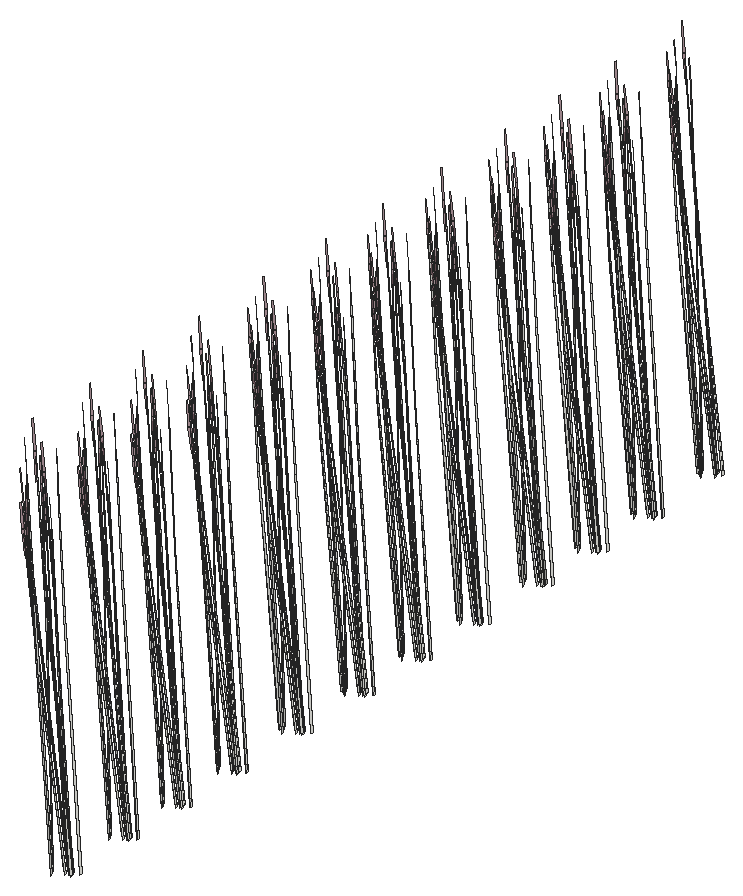
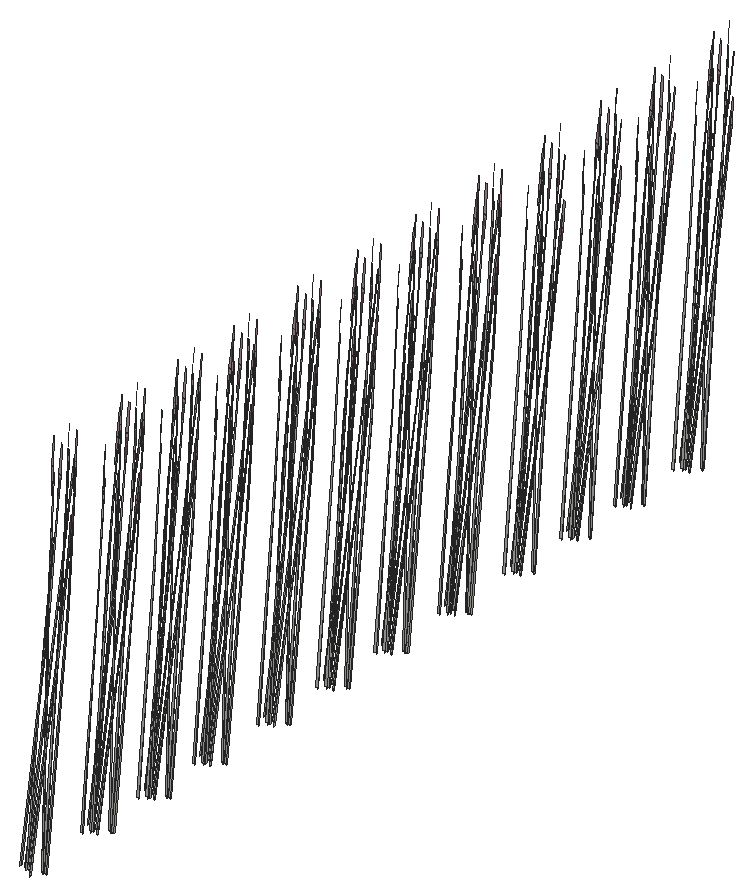
# SketchUp Ruby script. Lengths in inches.
U = 1.inch
M = Sketchup.active_model
def pt(a) = Geom::Point3d.new(a.map { |v| v * U })
def face(e, loops, mat)
  f = e.add_face(loops[0].map { |a| pt(a) })
  loops[1..].each { |l| e.add_face(l.map { |a| pt(a) }).erase! }
  f.material = f.back_material = mat if mat
  f
end
# faces: each face lists its corners as indices into pts; further lists are holes
def faces(e, pts, list, mat = nil) = list.each { |f| face(e, (f[0].is_a?(Array) ? f : [f]).map { |l| l.map { |i| pts[i] } }, mat) }
# xy, xz, yz: faces in a plane at the given z, y or x. An outline is a flat list of corners, or four numbers for a rectangle; further outlines are holes
def ring(l) = l.size == 4 ? [[l[0], l[1]], [l[2], l[1]], [l[2], l[3]], [l[0], l[3]]] : l.each_slice(2).to_a
def flat(e, list, mat, &to3) = list.each { |f| face(e, (f[0].is_a?(Array) ? f : [f]).map { |l| ring(l).map { |u, v| to3.(u, v) } }, mat) }
def xy(e, z, list, mat = nil) = flat(e, list, mat) { |x, y| [x, y, z] }
def xz(e, y, list, mat = nil) = flat(e, list, mat) { |x, z| [x, y, z] }
def yz(e, x, list, mat = nil) = flat(e, list, mat) { |y, z| [x, y, z] }
def lines(e, pts, list) = list.each { |a, b| e.add_line(pt(pts[a]), pt(pts[b])) }
# prism: a flat outline (further loops are holes) pulled along v
def prism(e, loops, v, mat = nil)
  f = face(e, loops, mat); d = Geom::Vector3d.new(v.map { |x| x * U })
  f.pushpull(f.normal.samedirection?(d) ? d.length : -d.length)
end
def box(e, o, s, mat = nil) = prism(e, [[o, [o[0] + s[0], o[1], o[2]], [o[0] + s[0], o[1] + s[1], o[2]], [o[0], o[1] + s[1], o[2]]]], [0, 0, s[2]], mat)
def at(x, y, z, deg = 0) = Geom::Transformation.translation(pt([x, y, z])) * Geom::Transformation.rotation(ORIGIN, Z_AXIS, deg.degrees)
def axes(o, x, y, z) = Geom::Transformation.new([*x, 0, *y, 0, *z, 0, *pt(o).to_a, 1])
def part(name) = M.definitions.add(name)
# library, detail: a bought-in or finely detailed component or shape, given as its bounding box
def library(name, o, s) = part(name).tap { |d| box(d.entities, o, s) }
def detail(e, o, s) = box(e.add_group.entities, o, s)
def put(e, d, t, mat = nil) = e.add_instance(d, t).tap { |i| i.material = mat if mat }
def group(e, t, mat = nil) = e.add_group.tap { |g| g.transformation = t; g.material = mat if mat }.entities
root = M.entities
M.materials.add("LightPink_Translucent").color = [144, 107, 117]
M.materials["LightPink_Translucent"].alpha = 0.75
c1 = part("blade")
p = [[2.15,0.21,22],[0,0.17,0],[0.09,0.45,0],[2.18,0.31,22],[2.29,0.31,22],[0.38,0.45,0],
  [2.48,0.24,33],[2.49,0.24,33],[2.48,0.22,33]]
faces(c1.entities,p,[[0,1,2,3],[4,5,2,3],[6,3,4,7],[8,0,3,6]])
c2 = part("seeds")
p = [[0.3,-0.1,1.38],[-0.01,-0.03,1.59],[-0.01,-0.03,0.03],[0.14,-0.07,-0.07],[0.29,-0.03,3],[0.15,0.01,3.11]]
faces(c2.entities,p,[[0,1,2,3],[1,0,4,5]],"LightPink_Translucent")
c3 = part("blade with seeds")
put(c3.entities,c1,at(0,0,0))
put(c3.entities,c2,axes([2.4,0.25,30.99],[1.5799,-0.05474,1.17369],[-0.12525,1.92788,0.29478],[-0.07173,-0.02425,1.56792]))
put(root,c3,axes([331.78,276.37,49.78],[0,-0.39075,-0.43871],[0.56491,0,0],[0,-0.089,1.3917]))
put(root,c3,axes([332.125,276.55,50.06],[-0.46965,0.32852,0.27176],[-0.46994,-0.32506,-0.32244],[-0.0164,-0.09329,1.45692]))
put(root,c3,axes([333.4,277.23,50.16],[0.13383,-0.46302,-0.20702],[0.63453,0.08071,0.45303],[-0.11087,-0.06394,1.38231]))
put(root,c3,axes([332.02,276.73,50.19],[0,0.39075,0.43871],[-0.56491,0,0],[0,-0.089,1.3917]))
put(root,c3,axes([333.35,277.05,49.95],[-0.30332,-0.32798,-0.39531],[0.45944,-0.23096,0.19025],[-0.09816,-0.04058,1.26923]))
put(root,c3,axes([332.52,277.77,49.79],[-0.11861,-0.34048,-0.27372],[0.47106,-0.09668,0.27372],[-0.09497,-0.03926,1.22797]))
put(root,c3,axes([333.63,277.34,50.3125],[-0.09741,0.34873,0.12794],[-0.4759,-0.06053,-0.36534],[-0.08661,-0.03581,1.11991]))
put(root,c3,axes([334.25,277.35,50.18],[-0.49304,-0.31451,-0.2226],[0.41487,-0.35316,0.48713],[-0.13277,0.03679,1.48635]))
put(root,c3,axes([332.95,277.95,50.19],[0.47255,0.19538,0.43871],[-0.28245,0.35034,0],[-0.10763,-0.0445,1.3917]))
put(root,c3,axes([334,277.28,49.95],[-0.54829,0.02412,-0.39531],[-0.04958,-0.40041,0.19025],[-0.09816,0.04058,1.26923]))
put(root,c3,axes([334.02,277.51,49.82],[-0.34009,0.2937,-0.55095],[-0.42248,-0.26632,-0.1446],[-0.13628,0.07327,1.21613]))
put(root,c3,axes([334.58,278.31,49.78],[-0.47255,0.19538,-0.43871],[-0.28245,-0.35034,0],[-0.10763,0.0445,1.3917]))
put(root,c3,axes([331.78,286.17,49.78],[0,-0.39075,-0.43871],[0.56491,0,0],[0,-0.089,1.3917]))
put(root,c3,axes([332.125,286.35,50.06],[-0.46965,0.32852,0.27176],[-0.46994,-0.32506,-0.32244],[-0.0164,-0.09329,1.45692]))
put(root,c3,axes([333.4,287.04,50.16],[0.13383,-0.46302,-0.20702],[0.63453,0.08071,0.45303],[-0.11087,-0.06394,1.38231]))
put(root,c3,axes([332.02,286.53,50.19],[0,0.39075,0.43871],[-0.56491,0,0],[0,-0.089,1.3917]))
put(root,c3,axes([333.35,286.85,49.95],[-0.30332,-0.32798,-0.39531],[0.45944,-0.23096,0.19025],[-0.09816,-0.04058,1.26923]))
put(root,c3,axes([332.52,287.58,49.79],[-0.11861,-0.34048,-0.27372],[0.47106,-0.09668,0.27372],[-0.09497,-0.03926,1.22797]))
put(root,c3,axes([333.63,287.15,50.3125],[-0.09741,0.34873,0.12794],[-0.4759,-0.06053,-0.36534],[-0.08661,-0.03581,1.11991]))
put(root,c3,axes([334.25,287.15,50.18],[-0.49304,-0.31451,-0.2226],[0.41487,-0.35316,0.48713],[-0.13277,0.03679,1.48635]))
put(root,c3,axes([332.95,287.75,50.19],[0.47255,0.19538,0.43871],[-0.28245,0.35034,0],[-0.10763,-0.0445,1.3917]))
put(root,c3,axes([334,287.08,49.95],[-0.54829,0.02412,-0.39531],[-0.04958,-0.40041,0.19025],[-0.09816,0.04058,1.26923]))
put(root,c3,axes([334.02,287.32,49.82],[-0.34009,0.2937,-0.55095],[-0.42248,-0.26632,-0.1446],[-0.13628,0.07327,1.21613]))
put(root,c3,axes([334.58,288.12,49.78],[-0.47255,0.19538,-0.43871],[-0.28245,-0.35034,0],[-0.10763,0.0445,1.3917]))
put(root,c3,axes([331.78,295.15,49.78],[0,-0.39075,-0.43871],[0.56491,0,0],[0,-0.089,1.3917]))
put(root,c3,axes([332.125,295.33,50.06],[-0.46965,0.32852,0.27176],[-0.46994,-0.32506,-0.32244],[-0.0164,-0.09329,1.45692]))
put(root,c3,axes([333.4,296.01,50.16],[0.13383,-0.46302,-0.20702],[0.63453,0.08071,0.45303],[-0.11087,-0.06394,1.38231]))
put(root,c3,axes([332.02,295.51,50.19],[0,0.39075,0.43871],[-0.56491,0,0],[0,-0.089,1.3917]))
put(root,c3,axes([333.35,295.82,49.95],[-0.30332,-0.32798,-0.39531],[0.45944,-0.23096,0.19025],[-0.09816,-0.04058,1.26923]))
put(root,c3,axes([332.52,296.55,49.79],[-0.11861,-0.34048,-0.27372],[0.47106,-0.09668,0.27372],[-0.09497,-0.03926,1.22797]))
put(root,c3,axes([333.63,296.12,50.3125],[-0.09741,0.34873,0.12794],[-0.4759,-0.06053,-0.36534],[-0.08661,-0.03581,1.11991]))
put(root,c3,axes([334.25,296.13,50.18],[-0.49304,-0.31451,-0.2226],[0.41487,-0.35316,0.48713],[-0.13277,0.03679,1.48635]))
put(root,c3,axes([332.95,296.73,50.19],[0.47255,0.19538,0.43871],[-0.28245,0.35034,0],[-0.10763,-0.0445,1.3917]))
put(root,c3,axes([334,296.06,49.95],[-0.54829,0.02412,-0.39531],[-0.04958,-0.40041,0.19025],[-0.09816,0.04058,1.26923]))
put(root,c3,axes([334.02,296.29,49.82],[-0.34009,0.2937,-0.55095],[-0.42248,-0.26632,-0.1446],[-0.13628,0.07327,1.21613]))
put(root,c3,axes([334.58,297.09,49.78],[-0.47255,0.19538,-0.43871],[-0.28245,-0.35034,0],[-0.10763,0.0445,1.3917]))
put(root,c3,axes([331.78,304.63,49.78],[0,-0.39075,-0.43871],[0.56491,0,0],[0,-0.089,1.3917]))
put(root,c3,axes([332.125,304.8125,50.06],[-0.46965,0.32852,0.27176],[-0.46994,-0.32506,-0.32244],[-0.0164,-0.09329,1.45692]))
put(root,c3,axes([333.4,305.5,50.16],[0.13383,-0.46302,-0.20702],[0.63453,0.08071,0.45303],[-0.11087,-0.06394,1.38231]))
put(root,c3,axes([332.02,304.99,50.19],[0,0.39075,0.43871],[-0.56491,0,0],[0,-0.089,1.3917]))
put(root,c3,axes([333.35,305.31,49.95],[-0.30332,-0.32798,-0.39531],[0.45944,-0.23096,0.19025],[-0.09816,-0.04058,1.26923]))
put(root,c3,axes([332.52,306.04,49.79],[-0.11861,-0.34048,-0.27372],[0.47106,-0.09668,0.27372],[-0.09497,-0.03926,1.22797]))
put(root,c3,axes([333.63,305.61,50.3125],[-0.09741,0.34873,0.12794],[-0.4759,-0.06053,-0.36534],[-0.08661,-0.03581,1.11991]))
put(root,c3,axes([334.25,305.61,50.18],[-0.49304,-0.31451,-0.2226],[0.41487,-0.35316,0.48713],[-0.13277,0.03679,1.48635]))
put(root,c3,axes([332.95,306.21,50.19],[0.47255,0.19538,0.43871],[-0.28245,0.35034,0],[-0.10763,-0.0445,1.3917]))
put(root,c3,axes([334,305.54,49.95],[-0.54829,0.02412,-0.39531],[-0.04958,-0.40041,0.19025],[-0.09816,0.04058,1.26923]))
put(root,c3,axes([334.02,305.78,49.82],[-0.34009,0.2937,-0.55095],[-0.42248,-0.26632,-0.1446],[-0.13628,0.07327,1.21613]))
put(root,c3,axes([334.58,306.58,49.78],[-0.47255,0.19538,-0.43871],[-0.28245,-0.35034,0],[-0.10763,0.0445,1.3917]))
put(root,c3,axes([331.78,315.62,49.78],[0,-0.39075,-0.43871],[0.56491,0,0],[0,-0.089,1.3917]))
put(root,c3,axes([331.64,315.92,50.1],[-0.63136,0,0],[0,-0.43672,-0.456],[0,-0.09947,1.44655]))
put(root,c3,axes([332.125,315.8,50.06],[-0.46965,0.32852,0.27176],[-0.46994,-0.32506,-0.32244],[-0.0164,-0.09329,1.45692]))
put(root,c3,axes([333.4,316.49,50.16],[0.13383,-0.46302,-0.20702],[0.63453,0.08071,0.45303],[-0.11087,-0.06394,1.38231]))
put(root,c3,axes([332.02,315.98,50.19],[0,0.39075,0.43871],[-0.56491,0,0],[0,-0.089,1.3917]))
put(root,c3,axes([333.35,316.3,49.95],[-0.30332,-0.32798,-0.39531],[0.45944,-0.23096,0.19025],[-0.09816,-0.04058,1.26923]))
put(root,c3,axes([332.52,317.03,49.79],[-0.11861,-0.34048,-0.27372],[0.47106,-0.09668,0.27372],[-0.09497,-0.03926,1.22797]))
put(root,c3,axes([333.63,316.6,50.3125],[-0.09741,0.34873,0.12794],[-0.4759,-0.06053,-0.36534],[-0.08661,-0.03581,1.11991]))
put(root,c3,axes([334.25,316.6,50.18],[-0.49304,-0.31451,-0.2226],[0.41487,-0.35316,0.48713],[-0.13277,0.03679,1.48635]))
put(root,c3,axes([332.95,317.2,50.19],[0.47255,0.19538,0.43871],[-0.28245,0.35034,0],[-0.10763,-0.0445,1.3917]))
put(root,c3,axes([334,316.53,49.95],[-0.54829,0.02412,-0.39531],[-0.04958,-0.40041,0.19025],[-0.09816,0.04058,1.26923]))
put(root,c3,axes([334.02,316.77,49.82],[-0.34009,0.2937,-0.55095],[-0.42248,-0.26632,-0.1446],[-0.13628,0.07327,1.21613]))
put(root,c3,axes([334.58,317.57,49.78],[-0.47255,0.19538,-0.43871],[-0.28245,-0.35034,0],[-0.10763,0.0445,1.3917]))
put(root,c3,axes([331.78,326.22,49.78],[0,-0.39075,-0.43871],[0.56491,0,0],[0,-0.089,1.3917]))
put(root,c3,axes([331.64,326.51,50.1],[-0.63136,0,0],[0,-0.43672,-0.456],[0,-0.09947,1.44655]))
put(root,c3,axes([332.125,326.4,50.06],[-0.46965,0.32852,0.27176],[-0.46994,-0.32506,-0.32244],[-0.0164,-0.09329,1.45692]))
put(root,c3,axes([333.4,327.08,50.16],[0.13383,-0.46302,-0.20702],[0.63453,0.08071,0.45303],[-0.11087,-0.06394,1.38231]))
put(root,c3,axes([332.02,326.58,50.19],[0,0.39075,0.43871],[-0.56491,0,0],[0,-0.089,1.3917]))
put(root,c3,axes([333.35,326.9,49.95],[-0.30332,-0.32798,-0.39531],[0.45944,-0.23096,0.19025],[-0.09816,-0.04058,1.26923]))
put(root,c3,axes([332.52,327.625,49.79],[-0.11861,-0.34048,-0.27372],[0.47106,-0.09668,0.27372],[-0.09497,-0.03926,1.22797]))
put(root,c3,axes([333.63,327.19,50.3125],[-0.09741,0.34873,0.12794],[-0.4759,-0.06053,-0.36534],[-0.08661,-0.03581,1.11991]))
put(root,c3,axes([334.25,327.2,50.18],[-0.49304,-0.31451,-0.2226],[0.41487,-0.35316,0.48713],[-0.13277,0.03679,1.48635]))
put(root,c3,axes([332.95,327.8,50.19],[0.47255,0.19538,0.43871],[-0.28245,0.35034,0],[-0.10763,-0.0445,1.3917]))
put(root,c3,axes([334,327.13,49.95],[-0.54829,0.02412,-0.39531],[-0.04958,-0.40041,0.19025],[-0.09816,0.04058,1.26923]))
put(root,c3,axes([334.02,327.36,49.82],[-0.34009,0.2937,-0.55095],[-0.42248,-0.26632,-0.1446],[-0.13628,0.07327,1.21613]))
put(root,c3,axes([334.58,328.16,49.78],[-0.47255,0.19538,-0.43871],[-0.28245,-0.35034,0],[-0.10763,0.0445,1.3917]))
put(root,c3,axes([331.78,335.92,49.78],[0,-0.39075,-0.43871],[0.56491,0,0],[0,-0.089,1.3917]))
put(root,c3,axes([331.64,336.22,50.1],[-0.63136,0,0],[0,-0.43672,-0.456],[0,-0.09947,1.44655]))
put(root,c3,axes([332.125,336.1,50.06],[-0.46965,0.32852,0.27176],[-0.46994,-0.32506,-0.32244],[-0.0164,-0.09329,1.45692]))
put(root,c3,axes([333.4,336.79,50.16],[0.13383,-0.46302,-0.20702],[0.63453,0.08071,0.45303],[-0.11087,-0.06394,1.38231]))
put(root,c3,axes([332.02,336.29,50.19],[0,0.39075,0.43871],[-0.56491,0,0],[0,-0.089,1.3917]))
put(root,c3,axes([333.35,336.6,49.95],[-0.30332,-0.32798,-0.39531],[0.45944,-0.23096,0.19025],[-0.09816,-0.04058,1.26923]))
put(root,c3,axes([332.52,337.33,49.79],[-0.11861,-0.34048,-0.27372],[0.47106,-0.09668,0.27372],[-0.09497,-0.03926,1.22797]))
put(root,c3,axes([333.63,336.9,50.3125],[-0.09741,0.34873,0.12794],[-0.4759,-0.06053,-0.36534],[-0.08661,-0.03581,1.11991]))
put(root,c3,axes([334.25,336.9,50.18],[-0.49304,-0.31451,-0.2226],[0.41487,-0.35316,0.48713],[-0.13277,0.03679,1.48635]))
put(root,c3,axes([332.95,337.51,50.19],[0.47255,0.19538,0.43871],[-0.28245,0.35034,0],[-0.10763,-0.0445,1.3917]))
put(root,c3,axes([334,336.84,49.95],[-0.54829,0.02412,-0.39531],[-0.04958,-0.40041,0.19025],[-0.09816,0.04058,1.26923]))
put(root,c3,axes([334.02,337.07,49.82],[-0.34009,0.2937,-0.55095],[-0.42248,-0.26632,-0.1446],[-0.13628,0.07327,1.21613]))
put(root,c3,axes([334.58,337.87,49.78],[-0.47255,0.19538,-0.43871],[-0.28245,-0.35034,0],[-0.10763,0.0445,1.3917]))
put(root,c3,axes([331.78,345.86,49.78],[0,-0.39075,-0.43871],[0.56491,0,0],[0,-0.089,1.3917]))
put(root,c3,axes([331.64,346.15,50.1],[-0.63136,0,0],[0,-0.43672,-0.456],[0,-0.09947,1.44655]))
put(root,c3,axes([332.125,346.04,50.06],[-0.46965,0.32852,0.27176],[-0.46994,-0.32506,-0.32244],[-0.0164,-0.09329,1.45692]))
put(root,c3,axes([333.4,346.72,50.16],[0.13383,-0.46302,-0.20702],[0.63453,0.08071,0.45303],[-0.11087,-0.06394,1.38231]))
put(root,c3,axes([332.02,346.22,50.19],[0,0.39075,0.43871],[-0.56491,0,0],[0,-0.089,1.3917]))
put(root,c3,axes([333.35,346.54,49.95],[-0.30332,-0.32798,-0.39531],[0.45944,-0.23096,0.19025],[-0.09816,-0.04058,1.26923]))
put(root,c3,axes([332.52,347.26,49.79],[-0.11861,-0.34048,-0.27372],[0.47106,-0.09668,0.27372],[-0.09497,-0.03926,1.22797]))
put(root,c3,axes([333.63,346.83,50.3125],[-0.09741,0.34873,0.12794],[-0.4759,-0.06053,-0.36534],[-0.08661,-0.03581,1.11991]))
put(root,c3,axes([334.25,346.84,50.18],[-0.49304,-0.31451,-0.2226],[0.41487,-0.35316,0.48713],[-0.13277,0.03679,1.48635]))
put(root,c3,axes([332.95,347.44,50.19],[0.47255,0.19538,0.43871],[-0.28245,0.35034,0],[-0.10763,-0.0445,1.3917]))
put(root,c3,axes([334,346.77,49.95],[-0.54829,0.02412,-0.39531],[-0.04958,-0.40041,0.19025],[-0.09816,0.04058,1.26923]))
put(root,c3,axes([334.02,347,49.82],[-0.34009,0.2937,-0.55095],[-0.42248,-0.26632,-0.1446],[-0.13628,0.07327,1.21613]))
put(root,c3,axes([334.58,347.8,49.78],[-0.47255,0.19538,-0.43871],[-0.28245,-0.35034,0],[-0.10763,0.0445,1.3917]))
put(root,c3,axes([331.78,356.58,49.78],[0,-0.39075,-0.43871],[0.56491,0,0],[0,-0.089,1.3917]))
put(root,c3,axes([331.64,356.875,50.1],[-0.63136,0,0],[0,-0.43672,-0.456],[0,-0.09947,1.44655]))
put(root,c3,axes([332.125,356.76,50.06],[-0.46965,0.32852,0.27176],[-0.46994,-0.32506,-0.32244],[-0.0164,-0.09329,1.45692]))
put(root,c3,axes([333.4,357.45,50.16],[0.13383,-0.46302,-0.20702],[0.63453,0.08071,0.45303],[-0.11087,-0.06394,1.38231]))
put(root,c3,axes([332.02,356.94,50.19],[0,0.39075,0.43871],[-0.56491,0,0],[0,-0.089,1.3917]))
put(root,c3,axes([333.35,357.26,49.95],[-0.30332,-0.32798,-0.39531],[0.45944,-0.23096,0.19025],[-0.09816,-0.04058,1.26923]))
put(root,c3,axes([332.52,357.99,49.79],[-0.11861,-0.34048,-0.27372],[0.47106,-0.09668,0.27372],[-0.09497,-0.03926,1.22797]))
put(root,c3,axes([333.63,357.56,50.3125],[-0.09741,0.34873,0.12794],[-0.4759,-0.06053,-0.36534],[-0.08661,-0.03581,1.11991]))
put(root,c3,axes([334.25,357.56,50.18],[-0.49304,-0.31451,-0.2226],[0.41487,-0.35316,0.48713],[-0.13277,0.03679,1.48635]))
put(root,c3,axes([332.95,358.16,50.19],[0.47255,0.19538,0.43871],[-0.28245,0.35034,0],[-0.10763,-0.0445,1.3917]))
put(root,c3,axes([334,357.49,49.95],[-0.54829,0.02412,-0.39531],[-0.04958,-0.40041,0.19025],[-0.09816,0.04058,1.26923]))
put(root,c3,axes([334.02,357.73,49.82],[-0.34009,0.2937,-0.55095],[-0.42248,-0.26632,-0.1446],[-0.13628,0.07327,1.21613]))
put(root,c3,axes([334.58,358.53,49.78],[-0.47255,0.19538,-0.43871],[-0.28245,-0.35034,0],[-0.10763,0.0445,1.3917]))
put(root,c3,axes([331.78,365.91,49.78],[0,-0.39075,-0.43871],[0.56491,0,0],[0,-0.089,1.3917]))
put(root,c3,axes([331.64,366.2,50.1],[-0.63136,0,0],[0,-0.43672,-0.456],[0,-0.09947,1.44655]))
put(root,c3,axes([332.125,366.09,50.06],[-0.46965,0.32852,0.27176],[-0.46994,-0.32506,-0.32244],[-0.0164,-0.09329,1.45692]))
put(root,c3,axes([333.4,366.77,50.16],[0.13383,-0.46302,-0.20702],[0.63453,0.08071,0.45303],[-0.11087,-0.06394,1.38231]))
put(root,c3,axes([332.02,366.27,50.19],[0,0.39075,0.43871],[-0.56491,0,0],[0,-0.089,1.3917]))
put(root,c3,axes([333.35,366.58,49.95],[-0.30332,-0.32798,-0.39531],[0.45944,-0.23096,0.19025],[-0.09816,-0.04058,1.26923]))
put(root,c3,axes([332.52,367.3125,49.79],[-0.11861,-0.34048,-0.27372],[0.47106,-0.09668,0.27372],[-0.09497,-0.03926,1.22797]))
put(root,c3,axes([333.63,366.88,50.3125],[-0.09741,0.34873,0.12794],[-0.4759,-0.06053,-0.36534],[-0.08661,-0.03581,1.11991]))
put(root,c3,axes([334.25,366.89,50.18],[-0.49304,-0.31451,-0.2226],[0.41487,-0.35316,0.48713],[-0.13277,0.03679,1.48635]))
put(root,c3,axes([332.95,367.49,50.19],[0.47255,0.19538,0.43871],[-0.28245,0.35034,0],[-0.10763,-0.0445,1.3917]))
put(root,c3,axes([334,366.82,49.95],[-0.54829,0.02412,-0.39531],[-0.04958,-0.40041,0.19025],[-0.09816,0.04058,1.26923]))
put(root,c3,axes([334.02,367.05,49.82],[-0.34009,0.2937,-0.55095],[-0.42248,-0.26632,-0.1446],[-0.13628,0.07327,1.21613]))
put(root,c3,axes([334.58,367.85,49.78],[-0.47255,0.19538,-0.43871],[-0.28245,-0.35034,0],[-0.10763,0.0445,1.3917]))
put(root,c3,axes([331.78,375.38,49.78],[0,-0.39075,-0.43871],[0.56491,0,0],[0,-0.089,1.3917]))
put(root,c3,axes([331.64,375.67,50.1],[-0.63136,0,0],[0,-0.43672,-0.456],[0,-0.09947,1.44655]))
put(root,c3,axes([332.125,375.56,50.06],[-0.46965,0.32852,0.27176],[-0.46994,-0.32506,-0.32244],[-0.0164,-0.09329,1.45692]))
put(root,c3,axes([333.4,376.24,50.16],[0.13383,-0.46302,-0.20702],[0.63453,0.08071,0.45303],[-0.11087,-0.06394,1.38231]))
put(root,c3,axes([332.02,375.74,50.19],[0,0.39075,0.43871],[-0.56491,0,0],[0,-0.089,1.3917]))
put(root,c3,axes([333.35,376.06,49.95],[-0.30332,-0.32798,-0.39531],[0.45944,-0.23096,0.19025],[-0.09816,-0.04058,1.26923]))
put(root,c3,axes([332.52,376.78,49.79],[-0.11861,-0.34048,-0.27372],[0.47106,-0.09668,0.27372],[-0.09497,-0.03926,1.22797]))
put(root,c3,axes([333.63,376.35,50.3125],[-0.09741,0.34873,0.12794],[-0.4759,-0.06053,-0.36534],[-0.08661,-0.03581,1.11991]))
put(root,c3,axes([334.25,376.36,50.18],[-0.49304,-0.31451,-0.2226],[0.41487,-0.35316,0.48713],[-0.13277,0.03679,1.48635]))
put(root,c3,axes([332.95,376.96,50.19],[0.47255,0.19538,0.43871],[-0.28245,0.35034,0],[-0.10763,-0.0445,1.3917]))
put(root,c3,axes([334,376.29,49.95],[-0.54829,0.02412,-0.39531],[-0.04958,-0.40041,0.19025],[-0.09816,0.04058,1.26923]))
put(root,c3,axes([334.02,376.52,49.82],[-0.34009,0.2937,-0.55095],[-0.42248,-0.26632,-0.1446],[-0.13628,0.07327,1.21613]))
put(root,c3,axes([334.58,377.32,49.78],[-0.47255,0.19538,-0.43871],[-0.28245,-0.35034,0],[-0.10763,0.0445,1.3917]))
put(root,c3,axes([331.78,386.6875,49.78],[0,-0.39075,-0.43871],[0.56491,0,0],[0,-0.089,1.3917]))
put(root,c3,axes([331.64,386.98,50.1],[-0.63136,0,0],[0,-0.43672,-0.456],[0,-0.09947,1.44655]))
put(root,c3,axes([332.125,386.87,50.06],[-0.46965,0.32852,0.27176],[-0.46994,-0.32506,-0.32244],[-0.0164,-0.09329,1.45692]))
put(root,c3,axes([333.4,387.55,50.16],[0.13383,-0.46302,-0.20702],[0.63453,0.08071,0.45303],[-0.11087,-0.06394,1.38231]))
put(root,c3,axes([332.02,387.05,50.19],[0,0.39075,0.43871],[-0.56491,0,0],[0,-0.089,1.3917]))
put(root,c3,axes([333.35,387.37,49.95],[-0.30332,-0.32798,-0.39531],[0.45944,-0.23096,0.19025],[-0.09816,-0.04058,1.26923]))
put(root,c3,axes([332.52,388.09,49.79],[-0.11861,-0.34048,-0.27372],[0.47106,-0.09668,0.27372],[-0.09497,-0.03926,1.22797]))
put(root,c3,axes([333.63,387.66,50.3125],[-0.09741,0.34873,0.12794],[-0.4759,-0.06053,-0.36534],[-0.08661,-0.03581,1.11991]))
put(root,c3,axes([334.25,387.67,50.18],[-0.49304,-0.31451,-0.2226],[0.41487,-0.35316,0.48713],[-0.13277,0.03679,1.48635]))
